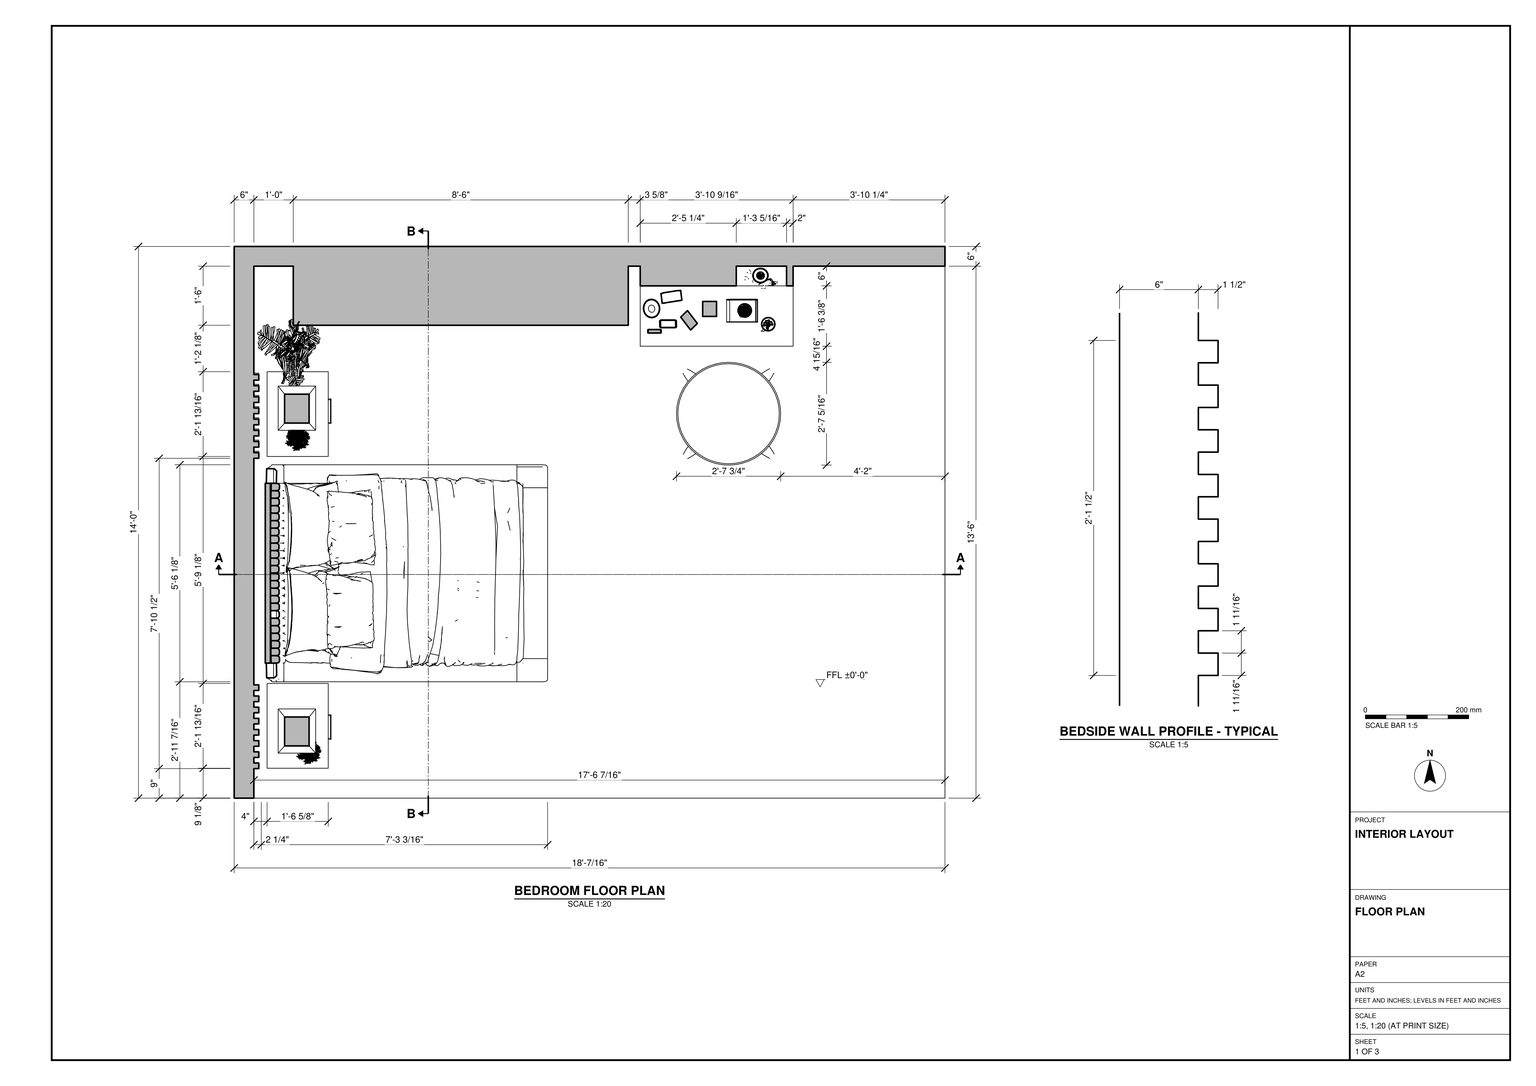
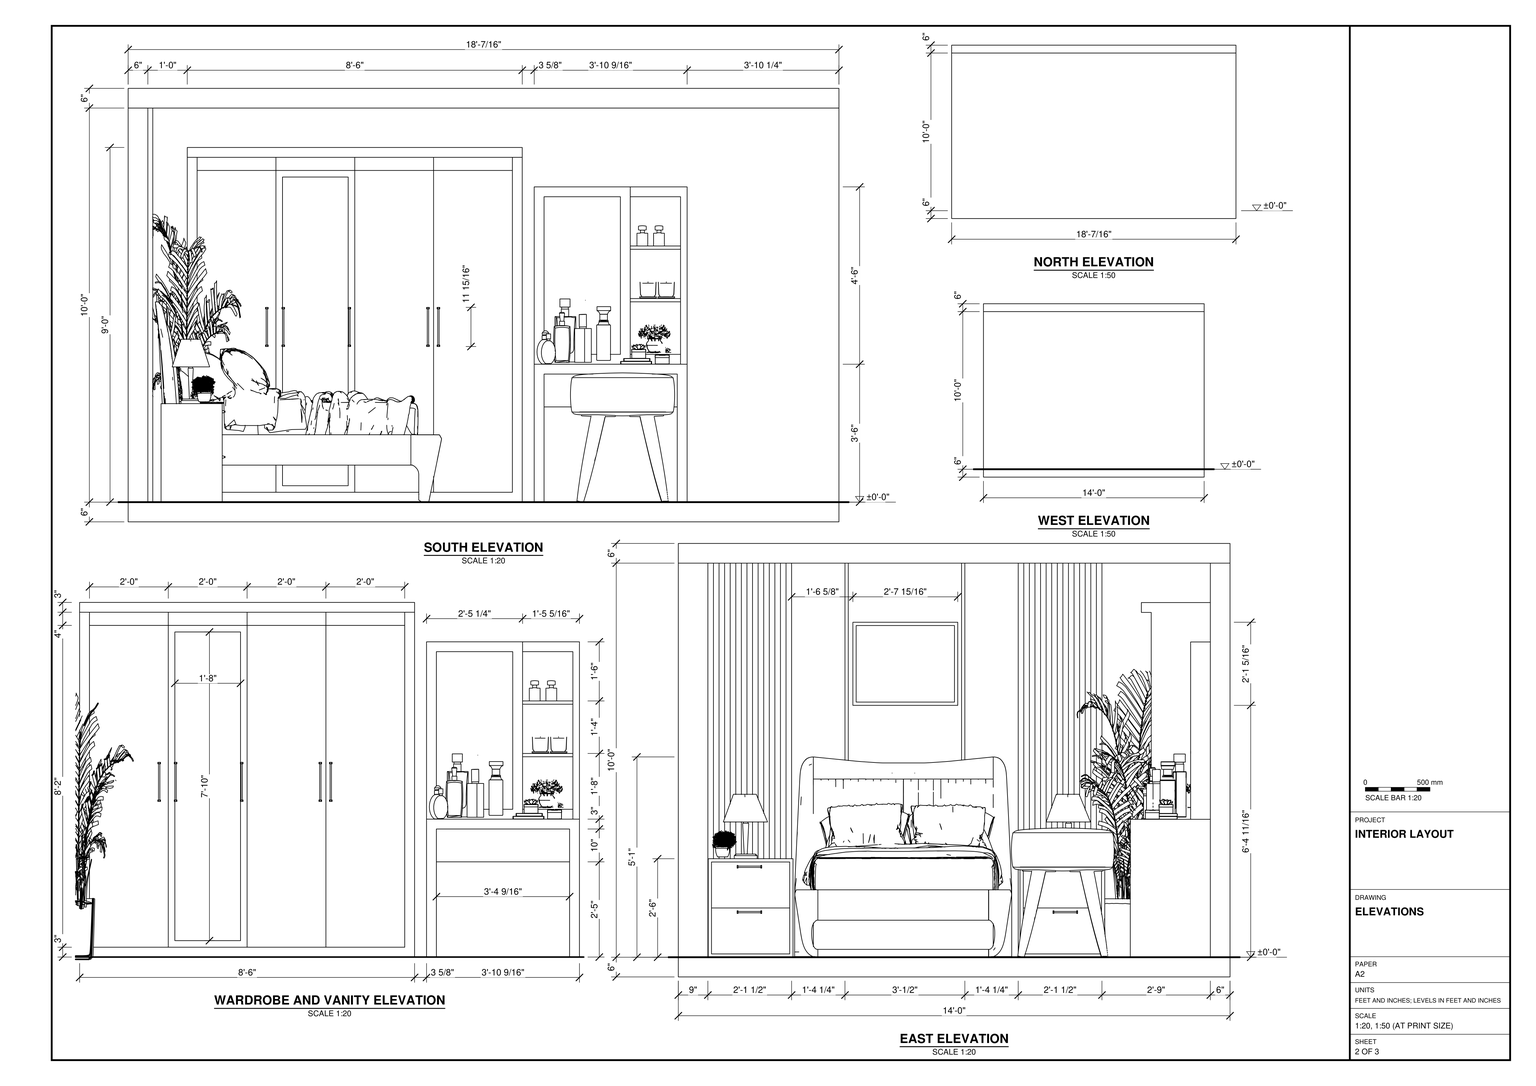
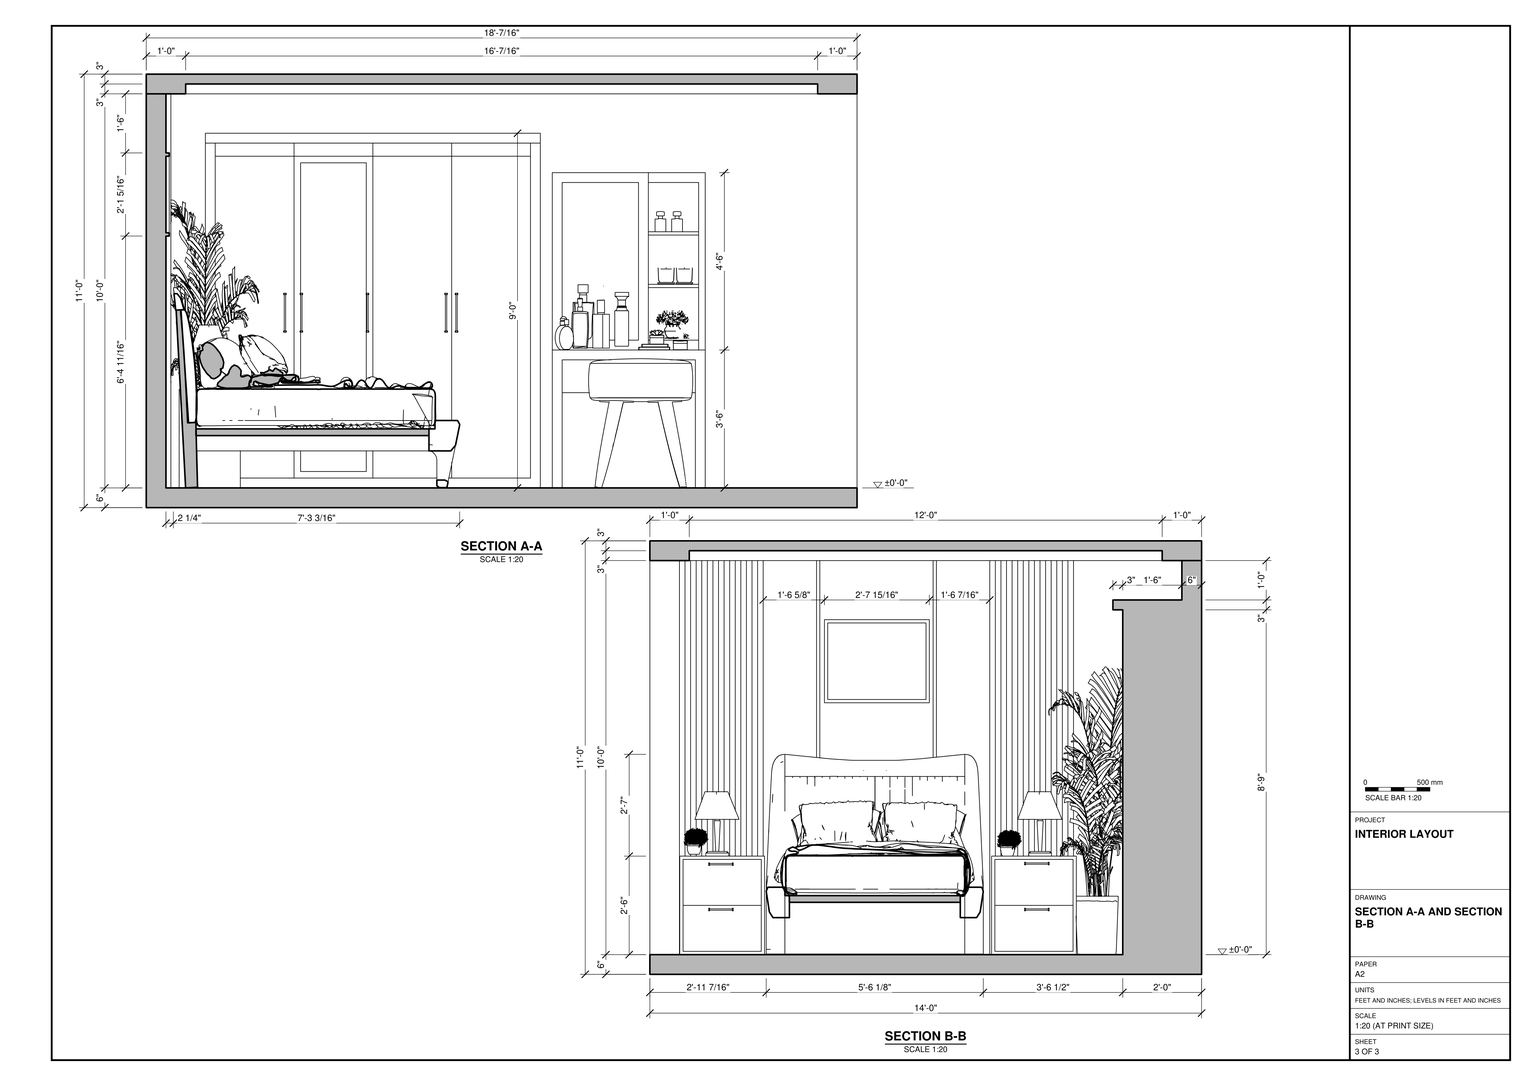
Build the bedroom in SketchUp from task_files/diagram_01.pdf. Work in feet and inches. The overall model extents are 18'-7/16" along X, 34'-7 7/16" along Y and 11'-0" along Z. For the bedroom itself, follow the 18'-7/16" by 14'-0" footprint on the floor plan. Set the finished floor at ±0'-0".

Model the 6" floor slab and the two adjoining 6" walls shown in plan. Use the sections to form the recessed ceiling, with its lower perimeter band 10'-0" above the finished floor. Place the bed with its headboard against the west wall and a drawer cabinet on either side. Detail the wall behind it with smooth panels, a rectangular frame above the headboard and projecting vertical ribs behind the cabinets. On the north wall, model the four-door wardrobe with its tall inset door panel. Place the vanity to its right, with a worktop, mirror, open shelves and a round stool in front.

Decor and loose items, including the bedside lamps, plants and objects on the vanity, may be any suitable library components. Keep the walls, slabs, ceiling and each furniture or joinery piece in separate groups or components, and use components for repeated parts. Save one SketchUp model as output_files/furnished_bedroom_with_a_wardrobe_and_vanity.skp.

# SketchUp Ruby script. Lengths in inches.
U = 1.inch
M = Sketchup.active_model
def pt(a) = Geom::Point3d.new(a.map { |v| v * U })
def face(e, loops, mat)
  f = e.add_face(loops[0].map { |a| pt(a) })
  loops[1..].each { |l| e.add_face(l.map { |a| pt(a) }).erase! }
  f.material = f.back_material = mat if mat
  f
end
# faces: each face lists its corners as indices into pts; further lists are holes
def faces(e, pts, list, mat = nil) = list.each { |f| face(e, (f[0].is_a?(Array) ? f : [f]).map { |l| l.map { |i| pts[i] } }, mat) }
# xy, xz, yz: faces in a plane at the given z, y or x. An outline is a flat list of corners, or four numbers for a rectangle; further outlines are holes
def ring(l) = l.size == 4 ? [[l[0], l[1]], [l[2], l[1]], [l[2], l[3]], [l[0], l[3]]] : l.each_slice(2).to_a
def flat(e, list, mat, &to3) = list.each { |f| face(e, (f[0].is_a?(Array) ? f : [f]).map { |l| ring(l).map { |u, v| to3.(u, v) } }, mat) }
def xy(e, z, list, mat = nil) = flat(e, list, mat) { |x, y| [x, y, z] }
def xz(e, y, list, mat = nil) = flat(e, list, mat) { |x, z| [x, y, z] }
def yz(e, x, list, mat = nil) = flat(e, list, mat) { |y, z| [x, y, z] }
def lines(e, pts, list) = list.each { |a, b| e.add_line(pt(pts[a]), pt(pts[b])) }
# prism: a flat outline (further loops are holes) pulled along v
def prism(e, loops, v, mat = nil)
  f = face(e, loops, mat); d = Geom::Vector3d.new(v.map { |x| x * U })
  f.pushpull(f.normal.samedirection?(d) ? d.length : -d.length)
end
def box(e, o, s, mat = nil) = prism(e, [[o, [o[0] + s[0], o[1], o[2]], [o[0] + s[0], o[1] + s[1], o[2]], [o[0], o[1] + s[1], o[2]]]], [0, 0, s[2]], mat)
def at(x, y, z, deg = 0) = Geom::Transformation.translation(pt([x, y, z])) * Geom::Transformation.rotation(ORIGIN, Z_AXIS, deg.degrees)
def axes(o, x, y, z) = Geom::Transformation.new([*x, 0, *y, 0, *z, 0, *pt(o).to_a, 1])
def part(name) = M.definitions.add(name)
# library, detail: a bought-in or finely detailed component or shape, given as its bounding box
def library(name, o, s) = part(name).tap { |d| box(d.entities, o, s) }
def detail(e, o, s) = box(e.add_group.entities, o, s)
def put(e, d, t, mat = nil) = e.add_instance(d, t).tap { |i| i.material = mat if mat }
def group(e, t, mat = nil) = e.add_group.tap { |g| g.transformation = t; g.material = mat if mat }.entities
root = M.entities
M.materials.add("[0045_Goldenrod]").color = [218, 165, 32]
M.materials.add("[0049_Beige]").color = [245, 245, 220]
M.materials.add("[Mirror 02]").color = [229, 229, 229]
M.materials.add("[Wood Veneer 01]").color = [120, 70, 37]
c1 = part("POI-E1497-320-1917\#1")
xy(c1.entities,0,[[0,0,0.29,0.83],[7.21,0,7.5,0.83]])
xy(c1.entities,0.64,[[0.29,0.21,7.21,0.62]])
xy(c1.entities,0.875,[[0,0.21,7.5,0.62]])
xz(c1.entities,0.21,[[0,0.64,7.5,0.875]])
xz(c1.entities,0.62,[[0,0.64,7.5,0.875]])
yz(c1.entities,0,[[0,0,0.21,0.64,0.21,0.875,0.62,0.875,0.62,0.64,0.83,0]])
yz(c1.entities,0.29,[[0,0,0.83,0,0.62,0.64,0.21,0.64]])
yz(c1.entities,7.21,[[0,0,0.21,0.64,0.62,0.64,0.83,0]])
yz(c1.entities,7.5,[[0,0,0.83,0,0.62,0.64,0.62,0.875,0.21,0.875,0.21,0.64]])
p = [[0,0.21,0.64],[0,0,0],[0.29,0,0],[0.29,0.21,0.64],[7.21,0.21,0.64],[7.21,0,0],
  [7.5,0,0],[7.5,0.21,0.64],[0,0.83,0],[0,0.62,0.64],[0.29,0.62,0.64],[0.29,0.83,0],
  [7.5,0.83,0],[7.5,0.62,0.64],[7.21,0.62,0.64],[7.21,0.83,0]]
faces(c1.entities,p,[[0,1,2,3],[4,5,6,7],[8,9,10,11],[12,13,14,15]])
c2 = library("LimeExp_giuong",[425.4,25.3,0.11],[85.56,94.09,41.21])
c3 = library("pleated+lamp",[-6.625,-6.625,0],[13.25,13.25,16.6875])
c4 = library("stool",[-0.68,-0.68,0],[1.36,1.36,1.75])
c5 = library("Table+Lamp",[-2.68,-8.73,0],[11.41,11.42,16.49])
c6 = library("suculentas com livro",[0,-0.27,0],[14.84,10.07,7.14])
c7 = library("Perfume bottle",[0,0,0],[3.29,1.23,4.58])
c8 = library("Candle",[-1.73,-1.73,0],[3.46,3.46,4.65])
c9 = library("parfumler",[1145.78,-651.38,138.39],[306.05,160.43,160.59])
c10 = library("N_Plant_4",[-12.12,-0.17,0],[15.33,15.33,4.43])
c11 = library("KentiaPalm",[-22.86,-14.31,0],[47.49,43.96,59.125])
c12 = library("Flower in vese",[-11.03,-2.08,0],[14.3,13.32,15.46])
xy(root,36,[[10.02,104.05,28.65,129.86]],"[Wood Veneer 01]")
xy(root,126,[[[0,0,216.4375,168],[12,12,204.4375,156]]],"[0049_Beige]")
xy(root,129,[[12,12,204.4375,156]],"[0049_Beige]")
xy(root,132,[[0,0,216.4375,168]],"[0049_Beige]")
xz(root,0,[[0,126,216.4375,132]],"[0049_Beige]")
xz(root,12,[[12,126,204.4375,129]],"[0049_Beige]")
xz(root,104.05,[[10.02,6,28.65,36]],"[Wood Veneer 01]")
xz(root,129.86,[[10.02,6,28.65,36]],"[Wood Veneer 01]")
xz(root,156,[[12,126,204.4375,129]],"[0049_Beige]")
xz(root,168,[[0,126,216.4375,132]],"[0049_Beige]")
yz(root,0,[[0,126,168,132]],"[0049_Beige]")
yz(root,10.02,[[104.05,6,129.86,36]],"[Wood Veneer 01]")
yz(root,12,[[12,126,156,129]],"[0049_Beige]")
yz(root,28.65,[[[104.05,6,129.86,36],[105.05,7,128.86,35]],[105.05,7,128.86,21],[105.05,21,128.86,35]],"[Wood Veneer 01]")
yz(root,204.4375,[[12,126,156,129]],"[0049_Beige]")
yz(root,216.4375,[[0,126,168,132]],"[0049_Beige]")
put(root,c1,axes([28.65,17.9,33.13],[0,1,0],[0,0,1],[1,0,0]))
put(root,c1,axes([28.65,17.9,19.32],[0,1,0],[0,0,1],[1,0,0]))
put(root,c1,axes([28.65,114.09,19.32],[0,1,0],[0,0,1],[1,0,0]))
put(root,c1,axes([28.65,114.09,33.32],[0,1,0],[0,0,1],[1,0,0]))
put(root,c2,axes([-15.1875,430.21,5.84],[0,-0.77264,0],[0.9266,0,0],[0,0,1.4803]))
put(root,c1,axes([41.82,144,65.31],[0,0,-1.59],[1,0,0],[0,-1,0]))
put(root,c1,axes([46.82,144,65.31],[0,0,-1.59],[1,0,0],[0,-1,0]))
put(root,c1,axes([66.94,144,65.31],[0,0,-1.59],[1,0,0],[0,-1,0]))
put(root,c1,axes([90.88,144,65.31],[0,0,-1.59],[1,0,0],[0,-1,0]))
put(root,c1,axes([94.07,144,65.31],[0,0,-1.59],[1,0,0],[0,-1,0]))
put(root,c3,at(68.04,408.84,0))
put(root,c4,axes([150.54,117.07,6.01],[23.4354,0,0],[0,23.11301,0],[0,0,22.47862]))
put(root,c5,axes([16.08,24,36],[1,0,0],[0,1.18,0],[0,0,1.19]))
put(root,c5,axes([16.08,122.3125,36],[1,0,0],[0,1.18,0],[0,0,1.19]))
put(root,c6,at(149.95,142.17,48))
put(root,c7,axes([154.93,157.08,84],[1,0,0],[0,1.82,0],[0,0,1.35]))
put(root,c8,axes([163.87,158.55,68],[1.4665,0,0],[0,1.4694,0],[0,0,1.41]))
put(root,c9,axes([40.54,195.21,30.87],[0.07328,0,0],[0,0.08255,0],[0,0,0.12379]))
put(root,c10,axes([28.21,4.94,36.55],[1.2,0,0],[0,1.2,0],[0,0,1.8]))
put(root,c10,axes([24.79,100.35,36],[1.2,0,0],[0,1.2,0],[0,0,1.8]))
put(root,c11,axes([17.37,132.66,5.31],[0.76,0,0],[0,1,0],[0,0,1.59778]))
put(root,c12,axes([163.11,156,51],[0.72,0,0],[0,0.69,0],[0,0,0.58]))
put(root,c8,axes([158.31,158.55,68],[1.4665,0,0],[0,1.4694,0],[0,0,1.41]))
put(root,c7,axes([159.99,157.08,84],[1,0,0],[0,1.82,0],[0,0,1.35]))
g1 = group(root,at(0,0,0),"[0049_Beige]")
xy(g1,0,[[0,0,216.4375,168]])
xy(g1,6,[[6,105.2,7.5,105.64],[6,108.6,7.5,109.04],[6,112,7.5,112.4375],[6,115.4,7.5,115.84],[6,118.8,7.5,119.24],
  [6,122.2,7.5,122.64],[6,125.6,7.5,126.04],[6,129,7.5,129.4375]])
xy(g1,6,[[[6,0,216.4375,0,216.4375,162,170.2,162,170.2,137.625,167.2,137.625,167.2,162,126.64,162,126.64,137.625,123.64,137.625,123.64,162,120,162,120,144,18,144,18,162,6,162,6,129.4375,7.5,129.4375,7.5,127.3,6,127.3,6,126.04,7.5,126.04,7.5,123.9,6,123.9,6,122.64,7.5,122.64,7.5,120.5,6,120.5,6,119.24,7.5,119.24,7.5,117.1,6,117.1,6,115.84,7.5,115.84,7.5,113.7,6,113.7,6,112.4375,7.5,112.4375,7.5,110.3,6,110.3,6,109.04,7.5,109.04,7.5,106.9,6,106.9,6,105.64,7.5,105.64,7.5,103.5,6,103.5,6,34.5,7.5,34.5,7.5,32.8,6,32.8,6,31.1,7.5,31.1,7.5,29.4,6,29.4,6,27.7,7.5,27.7,7.5,26,6,26,6,24.3,7.5,24.3,7.5,22.6,6,22.6,6,20.9,7.5,20.9,7.5,19.2,6,19.2,6,17.5,7.5,17.5,7.5,15.8,6,15.8,6,14.1,7.5,14.1,7.5,12.4,6,12.4,6,10.7,7.5,10.7,7.5,9,6,9],[10.02,9.11,28.65,34.92]]],"[0049_Beige]")
xy(g1,35,[[126.64,137.625,167.2,162]],"[Wood Veneer 01]")
xy(g1,36,[[10.02,9.11,28.65,34.92]],"[Wood Veneer 01]")
xy(g1,48,[[123.64,137.625,170.2,156]],"[Wood Veneer 01]")
xy(g1,51,[[152.89,156,168.2,162]],"[Wood Veneer 01]")
xy(g1,67,[[152.89,156,168.2,162]],"[Wood Veneer 01]")
xy(g1,68,[[152.89,156,168.2,162]],"[Wood Veneer 01]")
xy(g1,82.69,[[6,53.15,7,85.09]],"[Wood Veneer 01]")
xy(g1,83,[[152.89,156,168.2,162]],"[Wood Veneer 01]")
xy(g1,83.69,[[6,54.15,7,84.09]],"[Wood Veneer 01]")
xy(g1,84,[[152.89,156,168.2,162]],"[Wood Veneer 01]")
xy(g1,99,[[152.89,156,168.2,162]],"[Wood Veneer 01]")
xy(g1,102,[[123.64,156,170.2,162]],"[Wood Veneer 01]")
xy(g1,107.01,[[6,54.15,7,84.09]],"[Wood Veneer 01]")
xy(g1,108.01,[[6,53.15,7,85.09]],"[Wood Veneer 01]")
xy(g1,111,[[18,141,21,144],[21,141,45,144],[45,141,69,144],[69,141,93,144],[93,141,117,144],
  [117,141,120,144]],"[Wood Veneer 01]")
xy(g1,114,[[18,141,120,162]],"[Wood Veneer 01]")
xy(g1,126,[[0,0,6,0,6,9,7.5,9,7.5,10.7,6,10.7,6,12.4,7.5,12.4,7.5,14.1,6,14.1,6,15.8,7.5,15.8,7.5,17.5,6,17.5,6,19.2,7.5,19.2,7.5,20.9,6,20.9,6,22.6,7.5,22.6,7.5,24.3,6,24.3,6,26,7.5,26,7.5,27.7,6,27.7,6,29.4,7.5,29.4,7.5,31.1,6,31.1,6,32.8,7.5,32.8,7.5,34.5,6,34.5,6,103.5,7.5,103.5,7.5,105.2,6,105.2,6,106.9,7.5,106.9,7.5,108.6,6,108.6,6,110.3,7.5,110.3,7.5,112,6,112,6,113.7,7.5,113.7,7.5,115.4,6,115.4,6,117.1,7.5,117.1,7.5,118.8,6,118.8,6,120.5,7.5,120.5,7.5,122.2,6,122.2,6,123.9,7.5,123.9,7.5,125.6,6,125.6,6,127.3,7.5,127.3,7.5,129,6,129,6,168,0,168],[6,162,216.4375,168]])
xz(g1,0,[[0,0,216.4375,0,216.4375,6,6,6,6,126,0,126]])
xz(g1,9,[[6,6,7.5,126]],"[Wood Veneer 01]")
xz(g1,9.11,[[10.02,6,28.65,36]],"[Wood Veneer 01]")
xz(g1,10.7,[[6,6,7.5,126]],"[Wood Veneer 01]")
xz(g1,12.4,[[6,6,7.5,126]],"[Wood Veneer 01]")
xz(g1,14.1,[[6,6,7.5,126]],"[Wood Veneer 01]")
xz(g1,15.8,[[6,6,7.5,126]],"[Wood Veneer 01]")
xz(g1,17.5,[[6,6,7.5,126]],"[Wood Veneer 01]")
xz(g1,19.2,[[6,6,7.5,126]],"[Wood Veneer 01]")
xz(g1,20.9,[[6,6,7.5,126]],"[Wood Veneer 01]")
xz(g1,22.6,[[6,6,7.5,126]],"[Wood Veneer 01]")
xz(g1,24.3,[[6,6,7.5,126]],"[Wood Veneer 01]")
xz(g1,26,[[6,6,7.5,126]],"[Wood Veneer 01]")
xz(g1,27.7,[[6,6,7.5,126]],"[Wood Veneer 01]")
xz(g1,29.4,[[6,6,7.5,126]],"[Wood Veneer 01]")
xz(g1,31.1,[[6,6,7.5,126]],"[Wood Veneer 01]")
xz(g1,32.8,[[6,6,7.5,126]],"[Wood Veneer 01]")
xz(g1,34.5,[[6,6,7.5,126]],"[Wood Veneer 01]")
xz(g1,34.92,[[10.02,6,28.65,36]],"[Wood Veneer 01]")
xz(g1,53.15,[[6,82.69,7,108.01]],"[Wood Veneer 01]")
xz(g1,54.15,[[6,83.69,7,107.01]],"[Wood Veneer 01]")
xz(g1,84.09,[[6,83.69,7,107.01]],"[0049_Beige]")
xz(g1,85.09,[[6,82.69,7,108.01]],"[Wood Veneer 01]")
xz(g1,103.5,[[6,6,7.5,126]],"[Wood Veneer 01]")
xz(g1,105.2,[[6,6,7.5,126]],"[Wood Veneer 01]")
xz(g1,106.9,[[6,6,7.5,126]],"[Wood Veneer 01]")
xz(g1,108.6,[[6,6,7.5,126]],"[Wood Veneer 01]")
xz(g1,110.3,[[6,6,7.5,126]],"[Wood Veneer 01]")
xz(g1,112,[[6,6,7.5,126]],"[Wood Veneer 01]")
xz(g1,113.7,[[6,6,7.5,126]],"[Wood Veneer 01]")
xz(g1,115.4,[[6,6,7.5,126]],"[Wood Veneer 01]")
xz(g1,117.1,[[6,6,7.5,126]],"[Wood Veneer 01]")
xz(g1,118.8,[[6,6,7.5,126]],"[Wood Veneer 01]")
xz(g1,120.5,[[6,6,7.5,126]],"[Wood Veneer 01]")
xz(g1,122.2,[[6,6,7.5,126]],"[Wood Veneer 01]")
xz(g1,123.9,[[6,6,7.5,126]],"[Wood Veneer 01]")
xz(g1,125.6,[[6,6,7.5,126]],"[Wood Veneer 01]")
xz(g1,127.3,[[6,6,7.5,126]],"[Wood Veneer 01]")
xz(g1,129,[[6,6,7.5,126]],"[Wood Veneer 01]")
xz(g1,137.625,[[123.64,6,126.64,6,126.64,45,167.2,45,167.2,6,170.2,6,170.2,48,123.64,48],[126.64,35,167.2,45]],"[Wood Veneer 01]")
xz(g1,141,[[18,111,120,114]],"[Wood Veneer 01]")
xz(g1,144,[[47,11,67,105]],"[Mirror 02]")
xz(g1,144,[[18,6,120,6,120,111,117,111,117,9,21,9,21,111,18,111],[21,9,45,107],[[45,9,69,107],[47,11,67,105]],[69,9,93,107],[93,9,117,107],
  [21,107,45,111],[45,107,69,111],[69,107,93,111],[93,107,117,111]],"[Wood Veneer 01]")
xz(g1,156,[[126.64,51,149.89,99]],"[Mirror 02]")
xz(g1,156,[[[123.64,48,152.89,102],[126.64,51,149.89,99]],[152.89,48,168.2,51],[168.2,48,170.2,48,170.2,102,152.89,102,152.89,99,168.2,99],[152.89,67,168.2,68],[152.89,83,168.2,84]],"[Wood Veneer 01]")
xz(g1,162,[[6,6,18,6,18,114,120,114,120,6,123.64,6,123.64,102,170.2,102,170.2,6,216.4375,6,216.4375,126,6,126]],"[0049_Beige]")
xz(g1,162,[[126.64,6,167.2,35],[152.89,51,168.2,67],[152.89,68,168.2,83],[152.89,84,168.2,99]],"[Wood Veneer 01]")
xz(g1,168,[[0,0,216.4375,126]])
yz(g1,0,[[0,0,168,126]])
yz(g1,6,[[50.75,6,51.75,126],[86.25,6,87.25,126]],"[0045_Goldenrod]")
yz(g1,6,[[0,6,9,126],[34.5,6,50.75,126],[[51.75,6,86.25,126],[53.15,82.69,85.09,108.01]],[87.25,6,103.5,126],[129,6,162,126],
  [54.15,83.69,84.09,107.01]],"[0049_Beige]")
yz(g1,6,[[10.7,6,12.4,126],[14.1,6,15.8,126],[17.5,6,19.2,126],[20.9,6,22.6,126],[24.3,6,26,126],
  [27.7,6,29.4,126],[31.1,6,32.8,126],[105.2,6,106.9,126],[108.6,6,110.3,126],[112,6,113.7,126],
  [115.4,6,117.1,126],[118.8,6,120.5,126],[122.2,6,123.9,126],[125.6,6,127.3,126]],"[Wood Veneer 01]")
yz(g1,7,[[[53.15,82.69,85.09,108.01],[54.15,83.69,84.09,107.01]]],"[Wood Veneer 01]")
yz(g1,7.5,[[9,6,10.7,126],[12.4,6,14.1,126],[15.8,6,17.5,126],[19.2,6,20.9,126],[22.6,6,24.3,126],
  [26,6,27.7,126],[29.4,6,31.1,126],[32.8,6,34.5,126],[103.5,6,105.2,126],[106.9,6,108.6,126],
  [110.3,6,112,126],[113.7,6,115.4,126],[117.1,6,118.8,126],[120.5,6,122.2,126],[123.9,6,125.6,126],
  [127.3,6,129,126]],"[Wood Veneer 01]")
yz(g1,10.02,[[9.11,6,34.92,36]],"[Wood Veneer 01]")
yz(g1,18,[[144,6,144,111,141,111,141,114,162,114,162,6]],"[Wood Veneer 01]")
yz(g1,28.65,[[[9.11,6,34.92,36],[10.11,7,33.92,35]],[10.11,7,33.92,21],[10.11,21,33.92,35]],"[Wood Veneer 01]")
yz(g1,120,[[144,6,162,6,162,114,141,114,141,111,144,111]],"[Wood Veneer 01]")
yz(g1,123.64,[[137.625,6,162,48],[156,48,162,102]],"[Wood Veneer 01]")
yz(g1,126.64,[[137.625,6,162,35]],"[Wood Veneer 01]")
yz(g1,152.89,[[156,51,162,67],[156,68,162,83],[156,84,162,99]],"[Wood Veneer 01]")
yz(g1,167.2,[[137.625,6,162,35]],"[Wood Veneer 01]")
yz(g1,168.2,[[156,51,162,67],[156,68,162,83],[156,84,162,99]],"[Wood Veneer 01]")
yz(g1,170.2,[[137.625,6,162,48],[156,48,162,102]],"[Wood Veneer 01]")
yz(g1,216.4375,[[0,0,168,0,168,126,162,126,162,6,0,6]],"[0049_Beige]")
p = [[6,103.9375,6],[6,103.5,6],[6,110.74,6],[6,110.3,6],[6,117.54,6],[6,117.1,6],
  [6,120.9375,6],[6,120.5,6],[7.5,110.74,6],[6,127.74,6],[6,127.3,6],[6,124.34,6],
  [6,123.9,6],[6,107.34,6],[7.5,107.34,6],[7.5,103.9375,6],[6,114.14,6],[6,113.7,6],
  [6,106.9,6],[7.5,120.9375,6],[7.5,117.54,6],[7.5,127.74,6],[7.5,124.34,6],[7.5,114.14,6]]
lines(g1,p,[[0,1],[2,3],[4,5],[6,7],[2,8],[9,10],[11,12],[13,14],[0,15],[16,17],[13,18],[6,19],
  [4,20],[9,21],[11,22],[16,23]])
